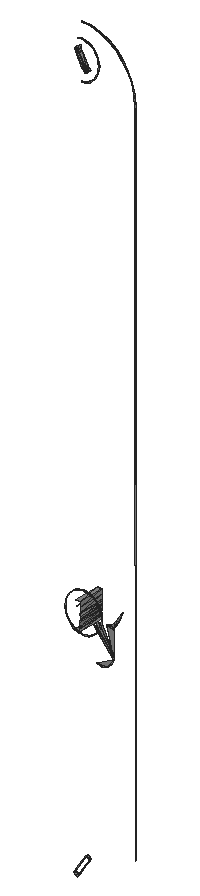
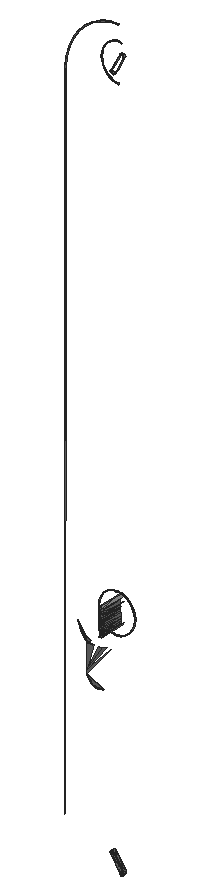
# SketchUp Ruby script. Lengths in inches.
U = 1.inch
M = Sketchup.active_model
def pt(a) = Geom::Point3d.new(a.map { |v| v * U })
def face(e, loops, mat)
  f = e.add_face(loops[0].map { |a| pt(a) })
  loops[1..].each { |l| e.add_face(l.map { |a| pt(a) }).erase! }
  f.material = f.back_material = mat if mat
  f
end
# faces: each face lists its corners as indices into pts; further lists are holes
def faces(e, pts, list, mat = nil) = list.each { |f| face(e, (f[0].is_a?(Array) ? f : [f]).map { |l| l.map { |i| pts[i] } }, mat) }
# xy, xz, yz: faces in a plane at the given z, y or x. An outline is a flat list of corners, or four numbers for a rectangle; further outlines are holes
def ring(l) = l.size == 4 ? [[l[0], l[1]], [l[2], l[1]], [l[2], l[3]], [l[0], l[3]]] : l.each_slice(2).to_a
def flat(e, list, mat, &to3) = list.each { |f| face(e, (f[0].is_a?(Array) ? f : [f]).map { |l| ring(l).map { |u, v| to3.(u, v) } }, mat) }
def xy(e, z, list, mat = nil) = flat(e, list, mat) { |x, y| [x, y, z] }
def xz(e, y, list, mat = nil) = flat(e, list, mat) { |x, z| [x, y, z] }
def yz(e, x, list, mat = nil) = flat(e, list, mat) { |y, z| [x, y, z] }
def lines(e, pts, list) = list.each { |a, b| e.add_line(pt(pts[a]), pt(pts[b])) }
# prism: a flat outline (further loops are holes) pulled along v
def prism(e, loops, v, mat = nil)
  f = face(e, loops, mat); d = Geom::Vector3d.new(v.map { |x| x * U })
  f.pushpull(f.normal.samedirection?(d) ? d.length : -d.length)
end
def box(e, o, s, mat = nil) = prism(e, [[o, [o[0] + s[0], o[1], o[2]], [o[0] + s[0], o[1] + s[1], o[2]], [o[0], o[1] + s[1], o[2]]]], [0, 0, s[2]], mat)
def at(x, y, z, deg = 0) = Geom::Transformation.translation(pt([x, y, z])) * Geom::Transformation.rotation(ORIGIN, Z_AXIS, deg.degrees)
def axes(o, x, y, z) = Geom::Transformation.new([*x, 0, *y, 0, *z, 0, *pt(o).to_a, 1])
def part(name) = M.definitions.add(name)
# library, detail: a bought-in or finely detailed component or shape, given as its bounding box
def library(name, o, s) = part(name).tap { |d| box(d.entities, o, s) }
def detail(e, o, s) = box(e.add_group.entities, o, s)
def put(e, d, t, mat = nil) = e.add_instance(d, t).tap { |i| i.material = mat if mat }
def group(e, t, mat = nil) = e.add_group.tap { |g| g.transformation = t; g.material = mat if mat }.entities
root = M.entities
M.materials.add("Material \#1").color = [140, 140, 140]
xy(root,40.525,[[109.178,196.69,109.209,196.69,109.209,197.002],[109.178,196.69,109.209,197.002,109.178,197.002]],"Material \#1")
xy(root,40.839,[[109.162,196.69,109.162,197.002,109.214,196.69],[109.214,196.69,109.162,197.002,109.214,197.002]],"Material \#1")
xz(root,196.734,[[109.82,38.331,109.809,46.173,109.809,44.483],[109.82,38.331,109.82,46.173,109.809,46.173],[109.809,46.173,109.82,46.173,109.799,46.299],[109.82,46.173,109.809,46.301,109.799,46.299],[109.188,46.224,109.224,46.24,109.188,46.236],
  [109.188,46.224,109.226,46.228,109.224,46.24],[109.226,46.228,109.257,46.25,109.224,46.24],[109.226,46.228,109.261,46.239,109.257,46.25],[109.261,46.239,109.288,46.266,109.257,46.25],[109.261,46.239,109.294,46.255,109.288,46.266],
  [109.294,46.255,109.316,46.287,109.288,46.266],[109.294,46.255,109.323,46.278,109.316,46.287],[109.323,46.278,109.34,46.313,109.316,46.287],[109.323,46.278,109.348,46.305,109.34,46.313],[109.799,46.299,109.809,46.301,109.77,46.413],
  [109.809,46.301,109.78,46.417,109.77,46.413],[109.348,46.305,109.36,46.343,109.34,46.313],[109.348,46.305,109.369,46.337,109.36,46.343],[109.369,46.337,109.375,46.377,109.36,46.343],[109.369,46.337,109.385,46.373,109.375,46.377],
  [109.385,46.373,109.384,46.414,109.375,46.377],[109.385,46.373,109.395,46.412,109.384,46.414],[109.395,46.412,109.387,46.452,109.384,46.414],[109.395,46.412,109.398,46.452,109.387,46.452],[109.77,46.413,109.78,46.417,109.724,46.518],
  [109.78,46.417,109.733,46.524,109.724,46.518],[109.387,46.452,109.398,46.452,109.384,46.491],[109.398,46.452,109.395,46.493,109.384,46.491],[109.384,46.491,109.395,46.493,109.375,46.528],[109.395,46.493,109.385,46.532,109.375,46.528],
  [109.724,46.518,109.733,46.524,109.663,46.612],[109.733,46.524,109.671,46.62,109.663,46.612],[109.375,46.528,109.385,46.532,109.36,46.561],[109.385,46.532,109.369,46.567,109.36,46.561],[109.36,46.561,109.369,46.567,109.34,46.592],
  [109.369,46.567,109.348,46.599,109.34,46.592],[109.34,46.592,109.348,46.599,109.316,46.618],[109.348,46.599,109.323,46.627,109.316,46.618],[109.663,46.612,109.671,46.62,109.588,46.694],[109.316,46.618,109.323,46.627,109.288,46.639],
  [109.671,46.62,109.595,46.703,109.588,46.694],[109.323,46.627,109.294,46.649,109.288,46.639],[109.288,46.639,109.294,46.649,109.257,46.655],[109.294,46.649,109.261,46.666,109.257,46.655],[109.257,46.655,109.261,46.666,109.224,46.665],
  [109.152,46.665,109.188,46.669,109.188,46.68],[109.224,46.665,109.226,46.677,109.188,46.669],[109.224,46.665,109.261,46.666,109.226,46.677],[109.188,46.669,109.226,46.677,109.188,46.68],[109.588,46.694,109.595,46.703,109.501,46.76],
  [109.595,46.703,109.507,46.77,109.501,46.76],[109.501,46.76,109.507,46.77,109.405,46.81],[109.507,46.77,109.408,46.821,109.405,46.81],[109.405,46.81,109.408,46.821,109.3,46.841],[109.408,46.821,109.302,46.853,109.3,46.841],
  [109.3,46.841,109.302,46.853,109.188,46.852],[109.188,46.852,109.302,46.853,109.188,46.864]],"Material \#1")
xz(root,196.767,[[109.188,40.447,109.188,40.455,109.132,40.455],[109.188,40.447,109.242,40.462,109.188,40.455],[109.188,40.447,109.244,40.455,109.242,40.462],[109.132,40.455,109.134,40.462,109.08,40.478],[109.132,40.455,109.188,40.455,109.134,40.462],
  [109.244,40.455,109.293,40.485,109.242,40.462],[109.244,40.455,109.296,40.478,109.293,40.485],[109.134,40.462,109.083,40.485,109.08,40.478],[109.08,40.478,109.083,40.485,109.035,40.516],[109.296,40.478,109.336,40.521,109.293,40.485],
  [109.296,40.478,109.341,40.516,109.336,40.521],[109.083,40.485,109.04,40.521,109.035,40.516],[109.035,40.516,109.04,40.521,109,40.564],[109.341,40.516,109.369,40.568,109.336,40.521],[109.341,40.516,109.376,40.564,109.369,40.568],
  [109.04,40.521,109.007,40.568,109,40.564],[109,40.564,109.007,40.568,108.979,40.621],[109.376,40.564,109.39,40.623,109.369,40.568],[109.376,40.564,109.397,40.621,109.39,40.623],[109.007,40.568,108.986,40.623,108.979,40.621],
  [108.979,40.621,108.986,40.623,108.971,40.682],[109.397,40.621,109.397,40.682,109.39,40.623],[109.397,40.621,109.405,40.682,109.397,40.682],[108.986,40.623,108.979,40.682,108.971,40.682],[108.971,40.682,108.979,40.682,108.979,40.743],
  [108.979,40.682,108.986,40.741,108.979,40.743],[109.397,40.682,109.405,40.682,109.39,40.741],[109.405,40.682,109.397,40.743,109.39,40.741],[108.986,40.741,109,40.8,108.979,40.743],[108.986,40.741,109.007,40.796,109,40.8],
  [109.39,40.741,109.397,40.743,109.369,40.796],[109.397,40.743,109.376,40.8,109.369,40.796],[109.007,40.796,109.035,40.849,109,40.8],[109.007,40.796,109.04,40.843,109.035,40.849],[109.369,40.796,109.376,40.8,109.336,40.843],
  [109.376,40.8,109.341,40.849,109.336,40.843],[109.04,40.843,109.08,40.886,109.035,40.849],[109.04,40.843,109.083,40.879,109.08,40.886],[109.336,40.843,109.341,40.849,109.293,40.879],[109.341,40.849,109.296,40.886,109.293,40.879],
  [109.083,40.879,109.132,40.91,109.08,40.886],[109.083,40.879,109.134,40.902,109.132,40.91],[109.293,40.879,109.296,40.886,109.242,40.902],[109.296,40.886,109.244,40.91,109.242,40.902],[109.134,40.902,109.188,40.918,109.132,40.91],
  [109.134,40.902,109.188,40.91,109.188,40.918],[109.242,40.902,109.244,40.91,109.188,40.91],[109.188,40.91,109.244,40.91,109.188,40.918]],"Material \#1")
xz(root,197.002,[[109.178,40.525,109.199,40.549,109.167,40.549],[109.178,40.525,109.209,40.525,109.199,40.549],[109.167,40.549,109.204,40.557,109.162,40.557],[109.167,40.549,109.199,40.549,109.204,40.557],[109.162,40.557,109.204,40.557,109.204,40.574],
  [109.162,40.557,109.204,40.574,109.162,40.574],[109.162,40.574,109.199,40.582,109.167,40.582],[109.162,40.574,109.204,40.574,109.199,40.582],[109.167,40.582,109.199,40.582,109.209,40.612],[109.167,40.582,109.209,40.612,109.167,40.612],
  [109.167,40.612,109.209,40.612,109.209,40.639],[109.167,40.612,109.209,40.639,109.167,40.639],[109.167,40.639,109.217,40.661,109.159,40.661],[109.167,40.639,109.209,40.639,109.217,40.661],[109.159,40.661,109.217,40.661,109.217,40.684],
  [109.159,40.661,109.217,40.684,109.159,40.684],[109.159,40.684,109.209,40.706,109.167,40.706],[109.159,40.684,109.217,40.684,109.209,40.706],[109.167,40.706,109.214,40.721,109.162,40.721],[109.167,40.706,109.209,40.706,109.214,40.721],
  [109.162,40.721,109.214,40.721,109.214,40.773],[109.162,40.721,109.214,40.773,109.162,40.773],[109.162,40.773,109.208,40.776,109.169,40.776],[109.162,40.773,109.214,40.773,109.208,40.776],[109.169,40.776,109.208,40.776,109.208,40.784],
  [109.169,40.776,109.208,40.784,109.169,40.784],[109.169,40.784,109.214,40.788,109.162,40.788],[109.169,40.784,109.208,40.784,109.214,40.788],[109.162,40.788,109.214,40.788,109.214,40.839],[109.162,40.788,109.214,40.839,109.162,40.839]],"Material \#1")
xz(root,197.036,[[109.188,40.003,109.128,40.018,109.248,40.018],[109.188,40.003,109.248,40.018,109.219,40.007],[109.128,40.018,109.322,40.118,109.248,40.018],[109.248,40.018,109.295,40.059,109.274,40.036],[109.248,40.018,109.322,40.118,109.295,40.059],
  [109.295,40.059,109.322,40.118,109.311,40.087],[109.322,40.118,109.046,40.46,109.325,40.152],[109.325,40.152,109.093,40.471,109.138,40.453],[109.325,40.152,109.138,40.453,109.188,40.447],[109.325,40.152,109.238,40.453,109.325,40.4375],
  [109.325,40.4375,109.238,40.453,109.327,40.45],[109.325,40.4375,109.327,40.45,109.326,40.444],[109.327,40.45,109.238,40.453,109.331,40.461],[109.327,40.45,109.331,40.461,109.328,40.456],[109.331,40.461,109.283,40.471,109.324,40.498],
  [109.331,40.461,109.324,40.498,109.357,40.535],[109.331,40.461,109.357,40.535,109.431,40.647],[109.331,40.461,109.431,40.647,109.334,40.466],[109.334,40.466,109.431,40.647,109.338,40.47],[109.338,40.47,109.384,40.524,109.342,40.475],
  [109.338,40.47,109.431,40.647,109.384,40.524],[109.342,40.475,109.384,40.524,109.364,40.498],[109.357,40.535,109.383,40.579,109.431,40.647]],"Material \#1")
yz(root,109.209,[[196.69,40.612,196.69,40.639,197.002,40.639],[196.69,40.612,197.002,40.639,197.002,40.612]],"Material \#1")
yz(root,109.214,[[196.69,40.721,197.002,40.773,197.002,40.721]],"Material \#1")
yz(root,109.217,[[196.69,40.661,196.69,40.684,197.002,40.684],[196.69,40.661,197.002,40.684,197.002,40.661]],"Material \#1")
p = [[109.1,196.741,37.962],[109.118,196.741,37.944],[109.118,196.767,37.944],[109.1,196.767,37.962],[109.14,196.741,37.931],[109.14,196.767,37.931],
  [109.156,196.733,37.956],[109.156,196.76,37.956],[109.206,196.73,38.127],[109.13,196.73,38.008],[109.13,196.757,38.008],[109.206,196.757,38.127],
  [109.116,196.733,37.986],[109.116,196.76,37.986],[109.17,196.73,37.978],[109.17,196.757,37.978],[109.246,196.73,38.097],[109.246,196.757,38.097],
  [109.261,196.733,38.118],[109.261,196.76,38.118],[109.236,196.741,38.173],[109.22,196.733,38.149],[109.22,196.76,38.149],[109.236,196.767,38.174],
  [109.276,196.741,38.143],[109.276,196.767,38.143],[109.258,196.741,38.161],[109.258,196.767,38.161],[109.209,196.69,40.525],[109.202,196.69,40.553],
  [109.199,197.002,40.549],[109.199,197.002,40.549],[109.209,197.002,40.525],[109.209,196.69,40.525],[109.202,196.69,40.553],[109.204,197.002,40.557],
  [109.199,197.002,40.549],[109.165,196.69,40.553],[109.178,196.69,40.525],[109.178,197.002,40.525],[109.167,197.002,40.549],[109.165,196.69,40.553],
  [109.202,196.69,40.578],[109.209,196.69,40.612],[109.209,197.002,40.612],[109.202,196.69,40.553],[109.202,196.69,40.578],[109.204,197.002,40.574],
  [109.204,197.002,40.557],[109.209,196.69,40.639],[109.217,196.69,40.661],[109.217,197.002,40.661],[109.209,197.002,40.639],[109.202,196.69,40.578],
  [109.199,197.002,40.582],[109.204,197.002,40.574],[109.209,197.002,40.612],[109.199,197.002,40.582],[109.202,196.69,40.578],[109.214,196.69,40.721],
  [109.212,196.69,40.782],[109.214,197.002,40.773],[109.209,196.69,40.706],[109.214,196.69,40.721],[109.214,197.002,40.721],[109.217,196.69,40.684],
  [109.209,196.69,40.706],[109.209,197.002,40.706],[109.214,197.002,40.721],[109.209,197.002,40.706],[109.209,196.69,40.706],[109.209,197.002,40.706],
  [109.217,197.002,40.684],[109.217,196.69,40.684],[109.212,196.69,40.782],[109.214,196.69,40.839],[109.214,197.002,40.839],[109.214,197.002,40.839],
  [109.214,197.002,40.788],[109.212,196.69,40.782],[109.212,196.69,40.782],[109.208,197.002,40.776],[109.214,197.002,40.773],[109.165,196.69,40.777],
  [109.169,197.002,40.776],[109.169,197.002,40.784],[109.165,196.69,40.777],[109.162,197.002,40.788],[109.165,196.69,40.777],[109.162,197.002,40.773],
  [109.212,196.69,40.782],[109.214,197.002,40.788],[109.208,197.002,40.784],[109.212,196.69,40.782],[109.213,196.733,46.353],[109.226,196.741,46.327],
  [109.226,196.767,46.327],[109.213,196.76,46.353],[109.249,196.741,46.337],[109.249,196.767,46.337],[109.269,196.741,46.354],[109.269,196.767,46.354],
  [109.134,196.73,46.502],[109.2,196.73,46.376],[109.2,196.757,46.376],[109.134,196.757,46.502],[109.255,196.733,46.38],[109.243,196.73,46.403],
  [109.243,196.757,46.403],[109.255,196.76,46.38],[109.176,196.73,46.528],[109.176,196.757,46.528],[109.107,196.741,46.551],[109.121,196.733,46.525],
  [109.121,196.76,46.525],[109.107,196.767,46.551],[109.164,196.733,46.552],[109.164,196.76,46.552],[109.15,196.741,46.578],[109.15,196.767,46.578],
  [109.127,196.741,46.567],[109.127,196.767,46.567]]
faces(root,p,[[0,1,2],[2,3,0],[1,4,5],[5,2,1],[4,6,7],[7,5,4],[8,9,10],[10,11,8],
  [9,12,13],[13,10,9],[12,0,3],[3,13,12],[6,14,15],[15,7,6],[14,16,17],[17,15,14],
  [16,18,19],[19,17,16],[20,21,22],[22,23,20],[21,8,11],[11,22,21],[18,24,25],[25,19,18],
  [24,26,27],[27,25,24],[26,20,23],[23,27,26],[28,29,30],[31,32,33],[34,35,36],[37,38,39],
  [39,40,41],[42,43,44],[45,46,47],[47,48,45],[49,50,51],[51,52,49],[53,54,55],[56,57,58],
  [59,60,61],[62,63,64],[65,66,67],[68,69,70],[71,72,73],[74,75,76],[77,78,79],[80,81,82],
  [83,84,85],[86,85,87],[88,89,84],[90,91,92],[93,92,81],[94,95,96],[96,97,94],[95,98,99],
  [99,96,95],[98,100,101],[101,99,98],[102,103,104],[104,105,102],[103,94,97],[97,104,103],[106,107,108],
  [108,109,106],[107,110,111],[111,108,107],[100,106,109],[109,101,100],[112,113,114],[114,115,112],[113,102,105],
  [105,114,113],[110,116,117],[117,111,110],[116,118,119],[119,117,116],[118,120,121],[121,119,118],[120,112,115],
  [115,121,120]],"Material \#1")
